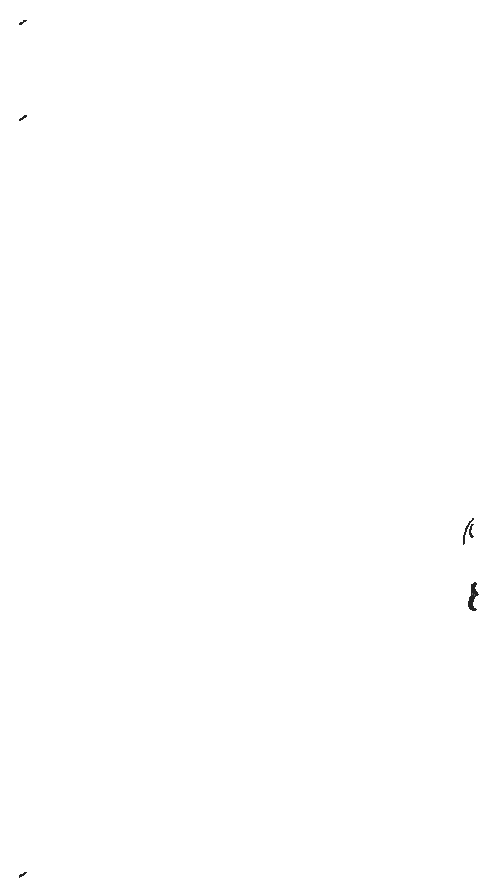
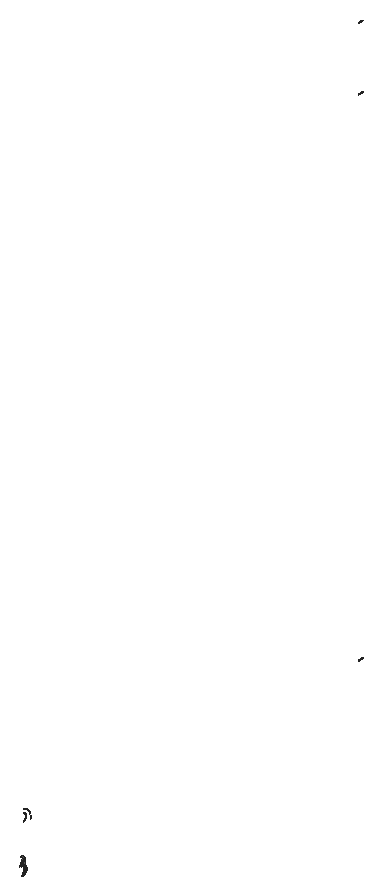
# SketchUp Ruby script. Lengths in inches.
U = 1.inch
M = Sketchup.active_model
def pt(a) = Geom::Point3d.new(a.map { |v| v * U })
def face(e, loops, mat)
  f = e.add_face(loops[0].map { |a| pt(a) })
  loops[1..].each { |l| e.add_face(l.map { |a| pt(a) }).erase! }
  f.material = f.back_material = mat if mat
  f
end
# faces: each face lists its corners as indices into pts; further lists are holes
def faces(e, pts, list, mat = nil) = list.each { |f| face(e, (f[0].is_a?(Array) ? f : [f]).map { |l| l.map { |i| pts[i] } }, mat) }
# xy, xz, yz: faces in a plane at the given z, y or x. An outline is a flat list of corners, or four numbers for a rectangle; further outlines are holes
def ring(l) = l.size == 4 ? [[l[0], l[1]], [l[2], l[1]], [l[2], l[3]], [l[0], l[3]]] : l.each_slice(2).to_a
def flat(e, list, mat, &to3) = list.each { |f| face(e, (f[0].is_a?(Array) ? f : [f]).map { |l| ring(l).map { |u, v| to3.(u, v) } }, mat) }
def xy(e, z, list, mat = nil) = flat(e, list, mat) { |x, y| [x, y, z] }
def xz(e, y, list, mat = nil) = flat(e, list, mat) { |x, z| [x, y, z] }
def yz(e, x, list, mat = nil) = flat(e, list, mat) { |y, z| [x, y, z] }
def lines(e, pts, list) = list.each { |a, b| e.add_line(pt(pts[a]), pt(pts[b])) }
# prism: a flat outline (further loops are holes) pulled along v
def prism(e, loops, v, mat = nil)
  f = face(e, loops, mat); d = Geom::Vector3d.new(v.map { |x| x * U })
  f.pushpull(f.normal.samedirection?(d) ? d.length : -d.length)
end
def box(e, o, s, mat = nil) = prism(e, [[o, [o[0] + s[0], o[1], o[2]], [o[0] + s[0], o[1] + s[1], o[2]], [o[0], o[1] + s[1], o[2]]]], [0, 0, s[2]], mat)
def at(x, y, z, deg = 0) = Geom::Transformation.translation(pt([x, y, z])) * Geom::Transformation.rotation(ORIGIN, Z_AXIS, deg.degrees)
def axes(o, x, y, z) = Geom::Transformation.new([*x, 0, *y, 0, *z, 0, *pt(o).to_a, 1])
def part(name) = M.definitions.add(name)
# library, detail: a bought-in or finely detailed component or shape, given as its bounding box
def library(name, o, s) = part(name).tap { |d| box(d.entities, o, s) }
def detail(e, o, s) = box(e.add_group.entities, o, s)
def put(e, d, t, mat = nil) = e.add_instance(d, t).tap { |i| i.material = mat if mat }
def group(e, t, mat = nil) = e.add_group.tap { |g| g.transformation = t; g.material = mat if mat }.entities
root = M.entities
M.materials.add("Material \#1").color = [140, 140, 140]
xy(root,58.0005,[[155.7326,414.0991,155.7283,414.11,155.7288,414.127],[155.7326,414.0991,155.7288,414.127,155.7326,414.1172],[155.7326,414.0991,155.7326,414.1172,155.7369,414.11],[155.7283,414.11,155.7245,414.1413,155.7253,414.1551],[155.7283,414.11,155.7253,414.1551,155.7288,414.127],
  [155.7369,414.11,155.7326,414.1172,155.7365,414.127],[155.7369,414.11,155.7365,414.127,155.7407,414.1413],[155.7365,414.127,155.7399,414.1551,155.7407,414.1413],[155.7245,414.1413,155.7217,414.1893,155.7228,414.1983],[155.7245,414.1413,155.7228,414.1983,155.7253,414.1551],
  [155.7407,414.1413,155.7399,414.1551,155.7435,414.1893],[155.7399,414.1551,155.7425,414.1983,155.7435,414.1893],[155.7217,414.1893,155.7202,414.2481,155.7215,414.2512],[155.7217,414.1893,155.7215,414.2512,155.7228,414.1983],[155.7435,414.1893,155.7425,414.1983,155.745,414.2481],
  [155.7425,414.1983,155.7438,414.2512,155.745,414.2481],[155.7202,414.2481,155.7202,414.3107,155.7215,414.3076],[155.7202,414.2481,155.7215,414.3076,155.7215,414.2512],[155.745,414.2481,155.7438,414.2512,155.745,414.3107],[155.7438,414.2512,155.7438,414.3076,155.745,414.3107],
  [155.7215,414.3076,155.7202,414.3107,155.7228,414.3605],[155.7438,414.3076,155.7425,414.3605,155.7435,414.3695],[155.7438,414.3076,155.7435,414.3695,155.745,414.3107],[155.7202,414.3107,155.7217,414.3695,155.7228,414.3605],[155.7228,414.3605,155.7217,414.3695,155.7253,414.4037],
  [155.7425,414.3605,155.7399,414.4037,155.7407,414.4175],[155.7425,414.3605,155.7407,414.4175,155.7435,414.3695],[155.7217,414.3695,155.7245,414.4175,155.7253,414.4037],[155.7253,414.4037,155.7245,414.4175,155.7288,414.4319],[155.7399,414.4037,155.7365,414.4319,155.7369,414.4488],
  [155.7399,414.4037,155.7369,414.4488,155.7407,414.4175],[155.7245,414.4175,155.7283,414.4488,155.7288,414.4319],[155.7288,414.4319,155.7283,414.4488,155.7326,414.4416],[155.7365,414.4319,155.7326,414.4416,155.7326,414.4597],[155.7365,414.4319,155.7326,414.4597,155.7369,414.4488],
  [155.7326,414.4416,155.7283,414.4488,155.7326,414.4597]],"Material \#1")
xy(root,58.0206,[[155.7326,414.0991,155.7326,414.1172,155.7283,414.11],[155.7326,414.0991,155.7365,414.127,155.7326,414.1172],[155.7326,414.0991,155.7369,414.11,155.7365,414.127],[155.7283,414.11,155.7288,414.127,155.7245,414.1413],[155.7283,414.11,155.7326,414.1172,155.7288,414.127],
  [155.7369,414.11,155.7399,414.1551,155.7365,414.127],[155.7369,414.11,155.7407,414.1413,155.7399,414.1551],[155.7288,414.127,155.7253,414.1551,155.7245,414.1413],[155.7245,414.1413,155.7253,414.1551,155.7217,414.1893],[155.7407,414.1413,155.7425,414.1983,155.7399,414.1551],
  [155.7407,414.1413,155.7435,414.1893,155.7425,414.1983],[155.7253,414.1551,155.7228,414.1983,155.7217,414.1893],[155.7217,414.1893,155.7228,414.1983,155.7202,414.2481],[155.7435,414.1893,155.7438,414.2512,155.7425,414.1983],[155.7435,414.1893,155.745,414.2481,155.7438,414.2512],
  [155.7228,414.1983,155.7215,414.2512,155.7202,414.2481],[155.7202,414.2481,155.7215,414.2512,155.7202,414.3107],[155.745,414.2481,155.7438,414.3076,155.7438,414.2512],[155.745,414.2481,155.745,414.3107,155.7438,414.3076],[155.7215,414.2512,155.7215,414.3076,155.7202,414.3107],
  [155.7215,414.3076,155.7217,414.3695,155.7202,414.3107],[155.7215,414.3076,155.7228,414.3605,155.7217,414.3695],[155.7438,414.3076,155.745,414.3107,155.7425,414.3605],[155.745,414.3107,155.7435,414.3695,155.7425,414.3605],[155.7228,414.3605,155.7245,414.4175,155.7217,414.3695],
  [155.7228,414.3605,155.7253,414.4037,155.7245,414.4175],[155.7425,414.3605,155.7435,414.3695,155.7399,414.4037],[155.7435,414.3695,155.7407,414.4175,155.7399,414.4037],[155.7253,414.4037,155.7283,414.4488,155.7245,414.4175],[155.7253,414.4037,155.7288,414.4319,155.7283,414.4488],
  [155.7399,414.4037,155.7407,414.4175,155.7365,414.4319],[155.7407,414.4175,155.7369,414.4488,155.7365,414.4319],[155.7288,414.4319,155.7326,414.4597,155.7283,414.4488],[155.7288,414.4319,155.7326,414.4416,155.7326,414.4597],[155.7365,414.4319,155.7369,414.4488,155.7326,414.4416],
  [155.7326,414.4416,155.7369,414.4488,155.7326,414.4597]],"Material \#1")
xy(root,93.6567,[[155.7326,414.0991,155.7283,414.11,155.7326,414.1172],[155.7326,414.0991,155.7326,414.1172,155.7365,414.127],[155.7326,414.0991,155.7365,414.127,155.7369,414.11],[155.7283,414.11,155.7245,414.1413,155.7288,414.127],[155.7283,414.11,155.7288,414.127,155.7326,414.1172],
  [155.7369,414.11,155.7365,414.127,155.7399,414.1551],[155.7369,414.11,155.7399,414.1551,155.7407,414.1413],[155.7288,414.127,155.7245,414.1413,155.7253,414.1551],[155.7245,414.1413,155.7217,414.1893,155.7253,414.1551],[155.7407,414.1413,155.7399,414.1551,155.7425,414.1983],
  [155.7407,414.1413,155.7425,414.1983,155.7435,414.1893],[155.7253,414.1551,155.7217,414.1893,155.7228,414.1983],[155.7217,414.1893,155.7202,414.2481,155.7228,414.1983],[155.7435,414.1893,155.7425,414.1983,155.7438,414.2512],[155.7435,414.1893,155.7438,414.2512,155.745,414.2481],
  [155.7228,414.1983,155.7202,414.2481,155.7215,414.2512],[155.7202,414.2481,155.7202,414.3107,155.7215,414.2512],[155.745,414.2481,155.7438,414.2512,155.7438,414.3076],[155.745,414.2481,155.7438,414.3076,155.745,414.3107],[155.7215,414.2512,155.7202,414.3107,155.7215,414.3076],
  [155.7215,414.3076,155.7202,414.3107,155.7217,414.3695],[155.7215,414.3076,155.7217,414.3695,155.7228,414.3605],[155.7438,414.3076,155.7425,414.3605,155.745,414.3107],[155.745,414.3107,155.7425,414.3605,155.7435,414.3695],[155.7228,414.3605,155.7217,414.3695,155.7245,414.4175],
  [155.7228,414.3605,155.7245,414.4175,155.7253,414.4037],[155.7425,414.3605,155.7399,414.4037,155.7435,414.3695],[155.7435,414.3695,155.7399,414.4037,155.7407,414.4175],[155.7253,414.4037,155.7245,414.4175,155.7283,414.4488],[155.7253,414.4037,155.7283,414.4488,155.7288,414.4319],
  [155.7399,414.4037,155.7365,414.4319,155.7407,414.4175],[155.7407,414.4175,155.7365,414.4319,155.7369,414.4488],[155.7288,414.4319,155.7283,414.4488,155.7326,414.4597],[155.7288,414.4319,155.7326,414.4597,155.7326,414.4416],[155.7365,414.4319,155.7326,414.4416,155.7369,414.4488],
  [155.7326,414.4416,155.7326,414.4597,155.7369,414.4488]],"Material \#1")
xy(root,93.6768,[[155.7326,414.0991,155.7288,414.127,155.7283,414.11],[155.7326,414.0991,155.7326,414.1172,155.7288,414.127],[155.7326,414.0991,155.7369,414.11,155.7326,414.1172],[155.7283,414.11,155.7253,414.1551,155.7245,414.1413],[155.7283,414.11,155.7288,414.127,155.7253,414.1551],
  [155.7369,414.11,155.7365,414.127,155.7326,414.1172],[155.7369,414.11,155.7407,414.1413,155.7365,414.127],[155.7365,414.127,155.7407,414.1413,155.7399,414.1551],[155.7245,414.1413,155.7228,414.1983,155.7217,414.1893],[155.7245,414.1413,155.7253,414.1551,155.7228,414.1983],
  [155.7407,414.1413,155.7435,414.1893,155.7399,414.1551],[155.7399,414.1551,155.7435,414.1893,155.7425,414.1983],[155.7217,414.1893,155.7215,414.2512,155.7202,414.2481],[155.7217,414.1893,155.7228,414.1983,155.7215,414.2512],[155.7435,414.1893,155.745,414.2481,155.7425,414.1983],
  [155.7425,414.1983,155.745,414.2481,155.7438,414.2512],[155.7202,414.2481,155.7215,414.2512,155.7215,414.3076],[155.7202,414.2481,155.7215,414.3076,155.7202,414.3107],[155.745,414.2481,155.745,414.3107,155.7438,414.2512],[155.7438,414.2512,155.745,414.3107,155.7438,414.3076],
  [155.7215,414.3076,155.7228,414.3605,155.7202,414.3107],[155.7438,414.3076,155.7435,414.3695,155.7425,414.3605],[155.7438,414.3076,155.745,414.3107,155.7435,414.3695],[155.7202,414.3107,155.7228,414.3605,155.7217,414.3695],[155.7228,414.3605,155.7253,414.4037,155.7217,414.3695],
  [155.7425,414.3605,155.7407,414.4175,155.7399,414.4037],[155.7425,414.3605,155.7435,414.3695,155.7407,414.4175],[155.7217,414.3695,155.7253,414.4037,155.7245,414.4175],[155.7253,414.4037,155.7288,414.4319,155.7245,414.4175],[155.7399,414.4037,155.7369,414.4488,155.7365,414.4319],
  [155.7399,414.4037,155.7407,414.4175,155.7369,414.4488],[155.7245,414.4175,155.7288,414.4319,155.7283,414.4488],[155.7288,414.4319,155.7326,414.4416,155.7283,414.4488],[155.7365,414.4319,155.7326,414.4597,155.7326,414.4416],[155.7365,414.4319,155.7369,414.4488,155.7326,414.4597],
  [155.7326,414.4416,155.7326,414.4597,155.7283,414.4488]],"Material \#1")
xy(root,98.1822,[[155.7326,414.0991,155.7283,414.11,155.7288,414.127],[155.7326,414.0991,155.7288,414.127,155.7326,414.1172],[155.7326,414.0991,155.7326,414.1172,155.7369,414.11],[155.7283,414.11,155.7245,414.1413,155.7253,414.1551],[155.7283,414.11,155.7253,414.1551,155.7288,414.127],
  [155.7369,414.11,155.7326,414.1172,155.7365,414.127],[155.7369,414.11,155.7365,414.127,155.7407,414.1413],[155.7365,414.127,155.7399,414.1551,155.7407,414.1413],[155.7245,414.1413,155.7217,414.1893,155.7228,414.1983],[155.7245,414.1413,155.7228,414.1983,155.7253,414.1551],
  [155.7407,414.1413,155.7399,414.1551,155.7435,414.1893],[155.7399,414.1551,155.7425,414.1983,155.7435,414.1893],[155.7217,414.1893,155.7202,414.2481,155.7215,414.2512],[155.7217,414.1893,155.7215,414.2512,155.7228,414.1983],[155.7435,414.1893,155.7425,414.1983,155.745,414.2481],
  [155.7425,414.1983,155.7438,414.2512,155.745,414.2481],[155.7202,414.2481,155.7202,414.3107,155.7215,414.3076],[155.7202,414.2481,155.7215,414.3076,155.7215,414.2512],[155.745,414.2481,155.7438,414.2512,155.745,414.3107],[155.7438,414.2512,155.7438,414.3076,155.745,414.3107],
  [155.7215,414.3076,155.7202,414.3107,155.7228,414.3605],[155.7438,414.3076,155.7425,414.3605,155.7435,414.3695],[155.7438,414.3076,155.7435,414.3695,155.745,414.3107],[155.7202,414.3107,155.7217,414.3695,155.7228,414.3605],[155.7228,414.3605,155.7217,414.3695,155.7253,414.4037],
  [155.7425,414.3605,155.7399,414.4037,155.7407,414.4175],[155.7425,414.3605,155.7407,414.4175,155.7435,414.3695],[155.7217,414.3695,155.7245,414.4175,155.7253,414.4037],[155.7253,414.4037,155.7245,414.4175,155.7288,414.4319],[155.7399,414.4037,155.7365,414.4319,155.7369,414.4488],
  [155.7399,414.4037,155.7369,414.4488,155.7407,414.4175],[155.7245,414.4175,155.7283,414.4488,155.7288,414.4319],[155.7288,414.4319,155.7283,414.4488,155.7326,414.4416],[155.7365,414.4319,155.7326,414.4416,155.7326,414.4597],[155.7365,414.4319,155.7326,414.4597,155.7369,414.4488],
  [155.7326,414.4416,155.7283,414.4488,155.7326,414.4597]],"Material \#1")
xy(root,98.2022,[[155.7326,414.0991,155.7365,414.127,155.7326,414.1172],[155.7326,414.0991,155.7369,414.11,155.7365,414.127],[155.7369,414.11,155.7399,414.1551,155.7365,414.127],[155.7369,414.11,155.7407,414.1413,155.7399,414.1551],[155.7407,414.1413,155.7425,414.1983,155.7399,414.1551],
  [155.7407,414.1413,155.7435,414.1893,155.7425,414.1983],[155.7435,414.1893,155.7438,414.2512,155.7425,414.1983],[155.7435,414.1893,155.745,414.2481,155.7438,414.2512],[155.745,414.2481,155.7438,414.3076,155.7438,414.2512],[155.745,414.2481,155.745,414.3107,155.7438,414.3076],
  [155.7438,414.3076,155.745,414.3107,155.7425,414.3605],[155.745,414.3107,155.7435,414.3695,155.7425,414.3605],[155.7425,414.3605,155.7435,414.3695,155.7399,414.4037],[155.7435,414.3695,155.7407,414.4175,155.7399,414.4037],[155.7399,414.4037,155.7407,414.4175,155.7365,414.4319],
  [155.7407,414.4175,155.7369,414.4488,155.7365,414.4319],[155.7365,414.4319,155.7369,414.4488,155.7326,414.4416],[155.7326,414.4416,155.7369,414.4488,155.7326,414.4597]],"Material \#1")
xy(root,98.2023,[[155.7283,414.11,155.7288,414.127,155.7245,414.1413],[155.7288,414.127,155.7253,414.1551,155.7245,414.1413],[155.7245,414.1413,155.7253,414.1551,155.7217,414.1893],[155.7253,414.1551,155.7228,414.1983,155.7217,414.1893],[155.7217,414.1893,155.7228,414.1983,155.7202,414.2481],
  [155.7228,414.1983,155.7215,414.2512,155.7202,414.2481],[155.7202,414.2481,155.7215,414.2512,155.7202,414.3107],[155.7215,414.2512,155.7215,414.3076,155.7202,414.3107],[155.7215,414.3076,155.7217,414.3695,155.7202,414.3107],[155.7215,414.3076,155.7228,414.3605,155.7217,414.3695],
  [155.7228,414.3605,155.7245,414.4175,155.7217,414.3695],[155.7228,414.3605,155.7253,414.4037,155.7245,414.4175],[155.7253,414.4037,155.7283,414.4488,155.7245,414.4175],[155.7253,414.4037,155.7288,414.4319,155.7283,414.4488]],"Material \#1")
yz(root,155.6343,[[444.0231,57.4405,443.8319,57.5685,443.9154,57.4752],[443.928,57.5113,443.8879,57.5469,443.8319,57.5685],[443.8879,57.5469,443.8544,57.5936,443.8319,57.5685],[443.8319,57.5685,443.7802,57.827,443.7845,57.7037],[443.8319,57.5685,443.8288,57.6495,443.7802,57.827],
  [443.8319,57.5685,443.7845,57.7037,443.8029,57.6319],[443.8319,57.5685,443.8544,57.5936,443.8288,57.6495],[443.8288,57.6495,443.8125,57.7129,443.7802,57.827],[443.7845,57.7037,443.7802,57.827,443.778,57.782],[443.8125,57.7129,443.8068,57.782,443.7802,57.827],
  [443.8068,57.782,443.8125,57.8511,443.7802,57.827],[443.7802,57.827,443.7969,57.9109,443.7866,57.87],[443.7802,57.827,443.8125,57.8511,443.8288,57.9145],[443.7802,57.827,443.8276,57.985,443.7969,57.9109],[443.7802,57.827,443.8288,57.9145,443.8806,58.0652],
  [443.7802,57.827,443.8738,58.0531,443.8276,57.985],[443.7969,57.9109,443.8276,57.985,443.8107,57.9493],[443.8276,57.985,443.8694,58.0475,443.8473,58.0178],[443.8276,57.985,443.8738,58.0531,443.8694,58.0475]],"Material \#1")
yz(root,155.6368,[[443.403,60.7893,443.4028,60.9536,443.3922,60.79],[443.403,60.7893,443.4134,60.9509,443.4028,60.9536],[443.9857,60.86,443.9876,60.8749,443.9501,60.8736],[443.9501,60.8736,443.9539,60.8878,443.9174,60.8953],[443.9501,60.8736,443.9876,60.8749,443.9539,60.8878],
  [443.9539,60.8878,443.9229,60.9083,443.9174,60.8953],[443.9174,60.8953,443.9229,60.9083,443.8882,60.9241],[443.9229,60.9083,443.8952,60.9356,443.8882,60.9241],[443.8882,60.9241,443.8952,60.9356,443.863,60.9592],[443.8952,60.9356,443.8713,60.9689,443.863,60.9592],
  [443.4134,60.9509,443.432,61.102,443.4028,60.9536],[443.4134,60.9509,443.4422,61.0967,443.432,61.102],[443.863,60.9592,443.8713,60.9689,443.8423,60.9999],[443.8713,60.9689,443.8517,61.0075,443.8423,60.9999],[443.8423,60.9999,443.8517,61.0075,443.8268,61.0455],
  [443.8517,61.0075,443.8369,61.0507,443.8268,61.0455],[443.8268,61.0455,443.8369,61.0507,443.817,61.095],[443.8369,61.0507,443.8277,61.0977,443.817,61.095],[443.817,61.095,443.8277,61.0977,443.8136,61.1472],[443.4422,61.0967,443.4787,61.2387,443.432,61.102],
  [443.4422,61.0967,443.488,61.2311,443.4787,61.2387],[443.8277,61.0977,443.8245,61.1472,443.8136,61.1472],[443.8136,61.1472,443.8245,61.1472,443.817,61.1994],[443.8245,61.1472,443.8277,61.1967,443.817,61.1994],[443.8277,61.1967,443.8268,61.2489,443.817,61.1994],
  [443.8277,61.1967,443.8369,61.2437,443.8268,61.2489],[443.488,61.2311,443.5409,61.3614,443.4787,61.2387],[443.488,61.2311,443.5492,61.3516,443.5409,61.3614],[443.8369,61.2437,443.8423,61.2945,443.8268,61.2489],[443.8369,61.2437,443.8517,61.2869,443.8423,61.2945],
  [443.8517,61.2869,443.863,61.3352,443.8423,61.2945],[443.8517,61.2869,443.8713,61.3255,443.863,61.3352],[443.8713,61.3255,443.8882,61.3703,443.863,61.3352],[443.8713,61.3255,443.8952,61.3588,443.8882,61.3703],[443.5492,61.3516,443.617,61.4674,443.5409,61.3614],
  [443.5492,61.3516,443.624,61.4558,443.617,61.4674],[443.8952,61.3588,443.9174,61.3991,443.8882,61.3703],[443.8952,61.3588,443.9229,61.3861,443.9174,61.3991],[443.9229,61.3861,443.9501,61.4208,443.9174,61.3991],[443.9229,61.3861,443.9539,61.4066,443.9501,61.4208],
  [443.9539,61.4066,443.9857,61.4344,443.9501,61.4208],[443.9539,61.4066,443.9876,61.4195,443.9857,61.4344],[443.624,61.4558,443.7051,61.5541,443.617,61.4674],[443.624,61.4558,443.7105,61.5411,443.7051,61.5541],[443.7105,61.5411,443.8032,61.6191,443.7051,61.5541],
  [443.7105,61.5411,443.807,61.6049,443.8032,61.6191],[443.807,61.6049,443.9097,61.6599,443.8032,61.6191],[443.807,61.6049,443.9117,61.645,443.9097,61.6599],[443.9117,61.645,444.0231,61.6741,443.9097,61.6599],[443.9117,61.645,444.0231,61.659,444.0231,61.6741]],"Material \#1")
yz(root,155.6595,[[444.0231,57.4405,443.8319,57.5685,443.928,57.5113],[444.0231,57.4405,443.9154,57.4752,443.8319,57.5685],[444.0231,57.4405,443.967,57.4495,443.9154,57.4752],[444.0231,57.4405,443.928,57.5113,443.9736,57.4886],[443.9154,57.4752,443.8698,57.5155,443.8319,57.5685],
  [443.928,57.5113,443.8319,57.5685,443.8879,57.5469],[443.8879,57.5469,443.8319,57.5685,443.8544,57.5936],[443.8319,57.5685,443.7802,57.827,443.8125,57.7129],[443.8319,57.5685,443.7845,57.7037,443.7802,57.827],[443.8319,57.5685,443.8029,57.6319,443.7845,57.7037],
  [443.8319,57.5685,443.8125,57.7129,443.8288,57.6495],[443.8319,57.5685,443.8288,57.6495,443.8544,57.5936],[443.7845,57.7037,443.778,57.782,443.7802,57.827],[443.8125,57.7129,443.7802,57.827,443.8068,57.782],[443.8068,57.782,443.7802,57.827,443.8125,57.8511],
  [443.7802,57.827,443.7866,57.87,443.7969,57.9109],[443.7802,57.827,443.7969,57.9109,443.8276,57.985],[443.7802,57.827,443.8276,57.985,443.8738,58.0531],[443.7802,57.827,443.8288,57.9145,443.8125,57.8511],[443.7802,57.827,443.8544,57.9704,443.8288,57.9145],
  [443.7802,57.827,443.8738,58.0531,443.8775,58.059],[443.7802,57.827,443.8775,58.059,443.8806,58.0652],[443.7802,57.827,443.8806,58.0652,443.8544,57.9704],[443.7969,57.9109,443.8107,57.9493,443.8276,57.985],[443.8544,57.9704,443.8806,58.0652,443.8879,58.0171],
  [443.8276,57.985,443.8473,58.0178,443.8694,58.0475],[443.8276,57.985,443.8694,58.0475,443.8738,58.0531],[443.8879,58.0171,443.8806,58.0652,443.928,58.0527],[443.928,58.0527,443.8806,58.0652,443.9736,58.0754],[443.8806,58.0652,443.883,58.0718,443.8847,58.0789],
  [443.8806,58.0652,443.8847,58.0789,443.9736,58.0754],[444.1654,58.0658,443.8861,58.46,443.8898,58.5038],[443.9736,58.0754,443.8847,58.0789,443.8861,58.0949],[443.9736,58.0754,443.8861,58.0949,443.8861,58.46],[443.9736,58.0754,443.8861,58.46,444.0231,58.0834],
  [443.8847,58.0789,443.8858,58.0866,443.8861,58.0949],[443.8898,58.5038,443.9001,58.5439,443.9163,58.5794],[443.8898,58.5038,443.9163,58.5794,443.9629,58.6315],[443.8898,58.5038,443.9629,58.6315,444.0834,58.6315],[443.9163,58.5794,443.9375,58.609,443.9629,58.6315]],"Material \#1")
yz(root,155.7604,[[444.0231,57.4405,443.8319,57.5685,443.9154,57.4752],[444.0231,57.4405,443.928,57.5113,443.8319,57.5685],[444.0231,57.4405,443.9154,57.4752,443.967,57.4495],[444.0231,57.4405,443.9736,57.4886,443.928,57.5113],[443.9154,57.4752,443.8319,57.5685,443.8698,57.5155],
  [443.928,57.5113,443.8879,57.5469,443.8319,57.5685],[443.8879,57.5469,443.8544,57.5936,443.8319,57.5685],[443.8319,57.5685,443.7802,57.827,443.7845,57.7037],[443.8319,57.5685,443.8125,57.7129,443.7802,57.827],[443.8319,57.5685,443.7845,57.7037,443.8029,57.6319],
  [443.8319,57.5685,443.8288,57.6495,443.8125,57.7129],[443.8319,57.5685,443.8544,57.5936,443.8288,57.6495],[443.7845,57.7037,443.7802,57.827,443.778,57.782],[443.8125,57.7129,443.8068,57.782,443.7802,57.827],[443.8068,57.782,443.8125,57.851,443.7802,57.827],
  [443.7802,57.827,443.7969,57.9109,443.7866,57.87],[443.7802,57.827,443.8125,57.851,443.8288,57.9145],[443.7802,57.827,443.8276,57.985,443.7969,57.9109],[443.7802,57.827,443.8288,57.9145,443.8544,57.9704],[443.7802,57.827,443.8544,57.9704,443.8806,58.0652],
  [443.7802,57.827,443.8738,58.0531,443.8276,57.985],[443.7802,57.827,443.8775,58.059,443.8738,58.0531],[443.7802,57.827,443.8806,58.0652,443.8775,58.059],[443.7969,57.9109,443.8276,57.985,443.8107,57.9493],[443.8544,57.9704,443.8879,58.0171,443.8806,58.0652],
  [443.8276,57.985,443.8694,58.0475,443.8473,58.0178],[443.8276,57.985,443.8738,58.0531,443.8694,58.0475],[443.8879,58.0171,443.928,58.0527,443.8806,58.0652],[443.928,58.0527,443.9736,58.0754,443.8806,58.0652],[443.8806,58.0652,443.8847,58.0789,443.883,58.0718],
  [443.8806,58.0652,443.9736,58.0754,443.8847,58.0789],[444.1654,58.0658,443.8898,58.5038,443.8861,58.46],[443.9736,58.0754,443.8861,58.0949,443.8847,58.0789],[443.9736,58.0754,443.8861,58.46,443.8861,58.0949],[443.9736,58.0754,444.0231,58.0834,443.8861,58.46],
  [443.8847,58.0789,443.8861,58.0949,443.8858,58.0866],[443.8898,58.5038,443.9163,58.5794,443.9001,58.5439],[443.8898,58.5038,443.9629,58.6315,443.9163,58.5794],[443.8898,58.5038,444.0834,58.6315,443.9629,58.6315],[443.9163,58.5794,443.9629,58.6315,443.9375,58.609],
  [443.9629,58.6315,444.0231,58.6509,443.9917,58.6459]],"Material \#1")
p = [[155.7283,414.11,98.2023],[155.7326,414.0991,98.2022],[155.7326,414.1172,98.2022],[155.7288,414.127,98.2023],[155.7326,414.4597,98.2022],[155.7283,414.4488,98.2023],
  [155.7288,414.4319,98.2023],[155.7326,414.4416,98.2022]]
faces(root,p,[[0,1,2],[2,3,0],[4,5,6],[6,7,4]],"Material \#1")
